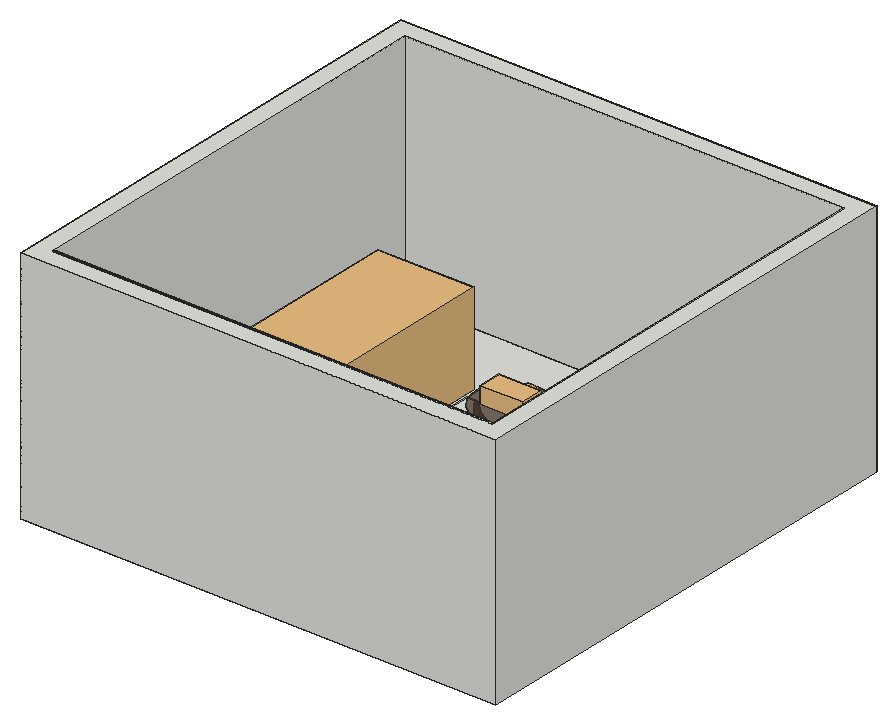
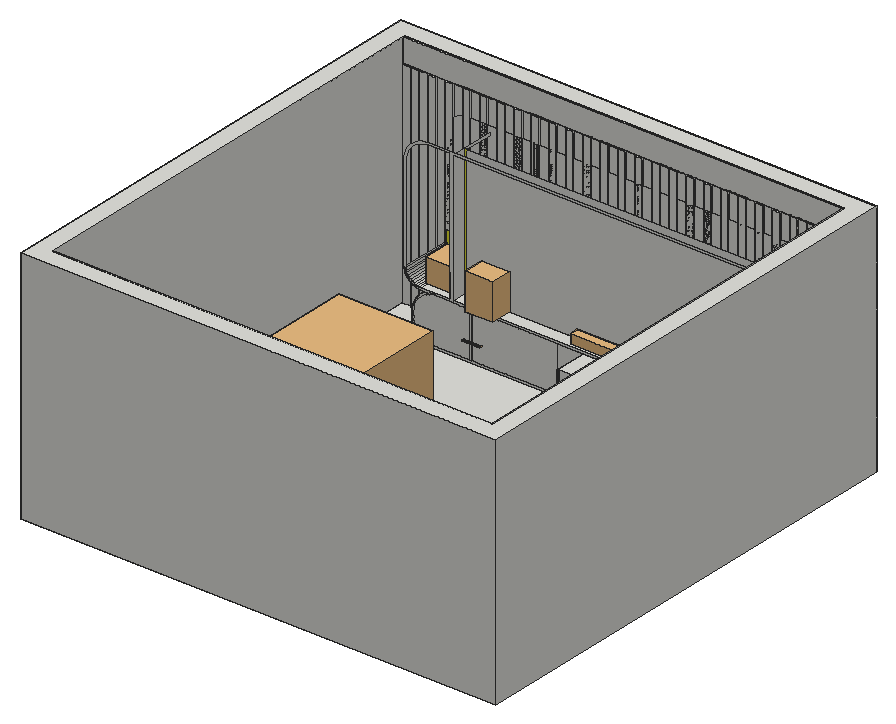
# SketchUp Ruby script. Lengths in inches.
U = 1.inch
M = Sketchup.active_model
def pt(a) = Geom::Point3d.new(a.map { |v| v * U })
def face(e, loops, mat)
  f = e.add_face(loops[0].map { |a| pt(a) })
  loops[1..].each { |l| e.add_face(l.map { |a| pt(a) }).erase! }
  f.material = f.back_material = mat if mat
  f
end
# faces: each face lists its corners as indices into pts; further lists are holes
def faces(e, pts, list, mat = nil) = list.each { |f| face(e, (f[0].is_a?(Array) ? f : [f]).map { |l| l.map { |i| pts[i] } }, mat) }
# xy, xz, yz: faces in a plane at the given z, y or x. An outline is a flat list of corners, or four numbers for a rectangle; further outlines are holes
def ring(l) = l.size == 4 ? [[l[0], l[1]], [l[2], l[1]], [l[2], l[3]], [l[0], l[3]]] : l.each_slice(2).to_a
def flat(e, list, mat, &to3) = list.each { |f| face(e, (f[0].is_a?(Array) ? f : [f]).map { |l| ring(l).map { |u, v| to3.(u, v) } }, mat) }
def xy(e, z, list, mat = nil) = flat(e, list, mat) { |x, y| [x, y, z] }
def xz(e, y, list, mat = nil) = flat(e, list, mat) { |x, z| [x, y, z] }
def yz(e, x, list, mat = nil) = flat(e, list, mat) { |y, z| [x, y, z] }
def lines(e, pts, list) = list.each { |a, b| e.add_line(pt(pts[a]), pt(pts[b])) }
# prism: a flat outline (further loops are holes) pulled along v
def prism(e, loops, v, mat = nil)
  f = face(e, loops, mat); d = Geom::Vector3d.new(v.map { |x| x * U })
  f.pushpull(f.normal.samedirection?(d) ? d.length : -d.length)
end
def box(e, o, s, mat = nil) = prism(e, [[o, [o[0] + s[0], o[1], o[2]], [o[0] + s[0], o[1] + s[1], o[2]], [o[0], o[1] + s[1], o[2]]]], [0, 0, s[2]], mat)
def at(x, y, z, deg = 0) = Geom::Transformation.translation(pt([x, y, z])) * Geom::Transformation.rotation(ORIGIN, Z_AXIS, deg.degrees)
def axes(o, x, y, z) = Geom::Transformation.new([*x, 0, *y, 0, *z, 0, *pt(o).to_a, 1])
def part(name) = M.definitions.add(name)
# library, detail: a bought-in or finely detailed component or shape, given as its bounding box
def library(name, o, s) = part(name).tap { |d| box(d.entities, o, s) }
def detail(e, o, s) = box(e.add_group.entities, o, s)
def put(e, d, t, mat = nil) = e.add_instance(d, t).tap { |i| i.material = mat if mat }
def group(e, t, mat = nil) = e.add_group.tap { |g| g.transformation = t; g.material = mat if mat }.entities
root = M.entities
M.materials.add("Color_D03").color = [255, 216, 101]
M.materials.add("Glass Dark").color = [71, 58, 43]
M.materials["Glass Dark"].alpha = 0.46
M.materials.add("[0134_DimGray]").color = [105, 105, 105]
M.materials.add("[0136_Charcoal]").color = [211, 185, 236]
M.materials.add("[Color G07]").color = [232, 230, 47]
M.materials.add("[Color M09]4").color = [0, 0, 0]
M.materials.add("notenhout").color = [99, 83, 84]
c1 = library("01",[0,0,0],[101.45,38.38,34.47])
c2 = library("Modern Round Tea Table",[0,0,0],[24.84,25.09,16.45])
c3 = part("Group\#19")
prism(c3.entities,[[[1.97,0,0],[1.97,39.37,0],[1.97,39.37,17.72],[1.97,37.14,17.72],[1.97,36.88,14.6875],[1.97,35.37,11.01],[1.97,32.79,7.79],[1.97,29.32,5.24],[1.97,25.19,3.54],[1.97,20.69,2.82],[1.97,16.12,3.1],[1.97,11.79,4.38],[1.97,8,6.58],[1.97,5.01,9.53],[1.97,3.01,13.03],[1.97,2.15,16.86],[1.97,2.23,17.72],[1.97,0,17.72]]],[-1.97,0,0],"notenhout")
c4 = part("japandi+table+glass+~")
g1 = group(c4.entities,at(26.82,84.01,17.85,-66.1))
prism(g1,[[[1.1875,15.62,0],[0,21.54,0],[0.38,27.57,0],[2.32,33.3,0],[5.67,38.33,0],[10.2,42.32,0],[15.62,45.01,0],[21.54,46.19,0],[27.57,45.81,0],[33.3,43.88,0],[38.33,40.53,0],[42.32,35.99,0],[45.01,30.58,0],[46.19,24.65,0],[45.81,18.62,0],[43.88,12.9,0],[40.53,7.86,0],[35.99,3.87,0],[30.58,1.1875,0],[24.65,0,0],[18.62,0.38,0],[12.9,2.32,0],[7.86,5.67,0],[3.87,10.2,0]]],[0,0,0.98],"Glass Dark")
put(c4.entities,c3,at(39.85,63.81,0,-66.1))
put(c4.entities,c3,at(50.43,90.37,0,-156.1))
c5 = part("232mm Slimline Handle")
detail(c5.entities,[0,0,0],[9.13,0.47,1.38])
c6 = part("skeF")
xy(c6.entities,0,[[0,0,50,36.34]])
xy(c6.entities,1.875,[[0,0,50,0,50,36.34,47.5,36.34,47.5,1.02,2.5,1.02,2.5,36.34,0,36.34]])
xy(c6.entities,2.8125,[[[2.5,1.02,47.5,6.25],[3.75,1.64,46.25,5.625]],[3.75,1.64,46.25,5.625]])
xy(c6.entities,3.75,[[[2.5,6.25,47.5,36.34],[5.625,9.375,44.375,33.125],[45.24,9.51,46.51,9.98],[45.24,11.8,46.51,12.27],[45.24,10.25,46.51,10.72],[45.24,10.99,46.51,11.46]],[5.625,9.375,44.375,33.125],[45.24,9.51,46.51,9.98],[45.24,10.25,46.51,10.72],[45.24,10.99,46.51,11.46],
  [45.24,11.8,46.51,12.27]])
xz(c6.entities,0,[[0,0,50,1.875]])
xz(c6.entities,1.02,[[2.5,1.875,47.5,2.8125]])
xz(c6.entities,6.25,[[2.5,2.8125,47.5,3.75]])
xz(c6.entities,36.34,[[0,0,50,1.875],[2.5,1.875,47.5,3.75]])
yz(c6.entities,0,[[0,0,36.34,1.875]])
yz(c6.entities,2.5,[[1.02,1.875,1.02,2.8125,6.25,2.8125,6.25,3.75,36.34,3.75,36.34,1.875]])
yz(c6.entities,47.5,[[1.02,1.875,36.34,1.875,36.34,3.75,6.25,3.75,6.25,2.8125,1.02,2.8125]])
yz(c6.entities,50,[[0,0,36.34,1.875]])
c7 = part("SONY\#1")
xy(c7.entities,0.02,[[1.44,0,1.15,0.02,0.9,0.07,0.68,0.16,0.51,0.28,0.375,0.43,0.27,0.6,0.21,0.79,0.19,1,0.5625,1,0.59,0.84,0.65,0.71,0.73,0.6,0.84,0.51,0.96,0.44,1.11,0.39,1.43,0.35,1.72,0.39,1.95,0.49,2.04,0.56,2.1,0.65,2.14,0.74,2.15,0.85,2.14,0.97,2.1,1.0625,2.04,1.14,1.95,1.21,1.67,1.32,1.23,1.43,0.8,1.55,0.64,1.63,0.51,1.72,0.41,1.83,0.34,1.95,0.3,2.08,0.29,2.23,0.31,2.4,0.36,2.56,0.45,2.7,0.57,2.82,0.73,2.92,0.91,2.99,1.11,3.04,1.34,3.05,1.57,3.04,1.79,2.99,1.98,2.92,2.14,2.82,2.28,2.69,2.375,2.54,2.4375,2.36,2.46,2.16,2.08,2.16,2.06,2.29,2.02,2.4,1.95,2.49,1.87,2.57,1.77,2.625,1.65,2.67,1.35,2.7,1.0625,2.67,0.85,2.58,0.77,2.51,0.71,2.43,0.68,2.35,0.67,2.25,0.7,2.09,0.8125,1.97,1.02,1.88,1.35,1.79,1.97,1.625,2.1875,1.52,2.37,1.36,2.44,1.26,2.49,1.15,2.52,1.03,2.54,0.88,2.52,0.7,2.46,0.54,2.36,0.39,2.23,0.25,2.07,0.14,1.88,0.0625,1.67,0.02],[[4.36,0,4.06,0.03,3.79,0.1,3.55,0.24,3.34,0.42,3.16,0.65,3.04,0.91,2.97,1.2,2.94,1.53,2.97,1.85,3.04,2.15,3.16,2.41,3.34,2.63,3.55,2.81,3.79,2.95,4.06,3.02,4.36,3.05,4.65,3.02,4.92,2.95,5.16,2.81,5.37,2.63,5.54,2.41,5.67,2.15,5.74,1.85,5.76,1.53,5.74,1.2,5.67,0.9,5.54,0.64,5.37,0.42,5.16,0.24,4.92,0.1,4.65,0.03],[4.35,0.33,4.5625,0.35,4.75,0.41,4.93,0.51,5.08,0.65,5.2,0.82,5.29,1.02,5.34,1.26,5.36,1.53,5.34,1.79,5.29,2.03,5.2,2.23,5.08,2.4,4.93,2.54,4.76,2.64,4.57,2.7,4.36,2.72,4.15,2.7,3.96,2.64,3.78,2.54,3.63,2.4,3.51,2.23,3.42,2.03,3.36,1.79,3.35,1.53,3.36,1.26,3.42,1.03,3.51,0.82,3.63,0.65,3.78,0.51,3.95,0.41,4.14,0.35]],[6.28,0.05,6.28,3,6.68,3,8.23,0.67,8.23,3,8.6,3,8.6,0.05,8.2,0.05,6.65,2.38,6.65,0.05],[10.11,0.05,10.11,1.3,8.95,3,9.42,3,10.31,1.64,11.18,3,11.66,3,10.5,1.3,10.5,0.05]])
c8 = part("Untitled (8)")
put(c8.entities,c6,at(36.34,-31.65,0),"Color_D03")
put(c8.entities,c7,at(55.46,-30.01,2.8125))
c9 = library("tasse",[17.31,42.26,0],[5.26,6.09,5.2])
c10 = library("Serving 10 ",[0,0,0],[18.76,10.8,8.42])
c11 = library("Panasonic+SC-HTB8+sound+bar",[0,-0.18,0],[29.53,4.33,2.36])
c12 = library("TV+remote",[138.89,58.58,0],[104.14,438.75,34])
c13 = library("Plant",[-15.17,-14.95,0],[35.27,31.45,46.14])
c14 = library("Buddha+++fountain+",[-17.29,-21.67,-1.59],[33.47,33.42,28.7])
c15 = library("Flower pot 12",[-12.91,-12.4,0],[25.81,25.8,45.6875])
xy(root,0,[[[0,0,240,240],[9,9,231,231]],[9,9,231,10],[[9,10,231,231],[76.664,81.343,148.977,185.781]],[13.856,11,204.943,12.6875]])
xy(root,0.1,[[76.664,81.343,148.977,185.781]])
xy(root,4,[[13.856,11,204.943,12.6875],[13.856,12.6875,204.943,37]])
xy(root,5,[[43.356,36.6,44.356,37],[87.051,36.6,88.051,36.788],[130.747,36.6,131.747,36.9],[174.443,36.6,175.443,37],[87.051,36.788,88.051,37],
  [130.747,36.9,131.747,37]])
xy(root,16.5,[[87.551,17,131.247,21],[87.551,21,88.051,36.6],[88.051,21,130.747,37],[130.747,21,131.247,36.6],[87.051,36.6,87.551,36.788],
  [87.551,36.6,88.051,36.788],[130.747,36.6,131.247,36.9],[131.247,36.6,131.747,36.9],[87.051,36.788,87.551,37],[131.247,36.9,131.747,37]])
xy(root,28,[[197.325,11,200.205,37],[87.551,17,131.247,21],[87.551,21,131.247,37],[43.356,36.6,44.356,37],[174.443,36.6,175.443,37]])
xy(root,29,[[26.356,11,204.189,11,204.189,37,200.205,37,200.205,11.1,185.773,11.1,185.773,37,183.773,37,183.773,30.3125,36.631,30.3125,36.631,26.3125,36.031,26.3125,36.031,30.3125,35.431,30.3125,35.431,26.3125,34.831,26.3125,34.831,30.3125,34.231,30.3125,34.231,26.3125,33.631,26.3125,33.631,30.3125,33.031,30.3125,33.031,26.3125,32.431,26.3125,32.431,30.3125,31.831,30.3125,31.831,26.3125,31.231,26.3125,31.231,30.3125,30.631,30.3125,30.631,26.3125,30.031,26.3125,30.031,30.3125,29.431,30.3125,29.431,26.375,28.831,26.375,28.831,30.3125,28.231,30.3125,28.231,26.375,27.631,26.375,27.631,30.3125,27.031,30.3125,27.031,26.375,26.431,26.375,26.431,30.3125,26.356,30.3125],[185.773,11.1,200.205,37],[24.079,15,24.231,30.3125],[30.031,26.3125,30.631,26.3125,30.631,30.3125,31.231,30.3125,31.231,26.3125,31.831,26.3125,31.831,30.3125,32.431,30.3125,32.431,26.3125,33.031,26.3125,33.031,30.3125,33.631,30.3125,33.631,26.3125,34.231,26.3125,34.231,30.3125,34.831,30.3125,34.831,26.3125,35.431,26.3125,35.431,30.3125,36.031,30.3125,36.031,26.3125,36.631,26.3125,36.631,30.3125,183.773,30.3125,183.773,37,24.079,37,24.079,30.3125,25.231,30.3125,25.231,26.375,25.831,26.375,25.831,30.3125,26.431,30.3125,26.431,26.375,27.031,26.375,27.031,30.3125,27.631,30.3125,27.631,26.375,28.231,26.375,28.231,30.3125,28.831,30.3125,28.831,26.375,29.431,26.375,29.431,30.3125,30.031,30.3125]])
xy(root,120,[[[0,0,240,240],[9,9,231,231]],[9,9,231,10]])
xz(root,0,[[0,0,240,120]])
xz(root,9,[[9,0,231,120]])
xz(root,10,[[13.856,0,13.856,108,9,108,9,120,231,120,231,0],[9,0,13.856,108]])
xz(root,11,[[13.856,0,204.943,4],[13.856,4,204.943,4,204.943,16.5,204.836,18.132,204.517,19.735,203.991,21.284,203.268,22.75,202.36,24.11,201.282,25.339,200.052,26.417,198.693,27.325,197.325,28,24.079,28,22.745,28.087,22.078,28.22,21.572,28.048,20.106,27.325,18.746,26.417,17.517,25.339,16.439,24.11,15.531,22.75,14.807,21.284,14.282,19.735,13.963,18.132,13.856,16.5],[13.856,16.5,13.856,29,19.717,29,20.167,28.778,21.433,28.348,22.078,28.22,21.572,28.048,20.106,27.325,18.746,26.417,17.517,25.339,16.439,24.11,15.531,22.75,14.807,21.284,14.282,19.735,13.963,18.132],[24.079,28,200.205,28,201.324,28.073,202.423,28.292,203.484,28.652,204.189,29,26.356,29,24.724,28.893,23.121,28.574,22.078,28.22,22.745,28.087],[22.078,28.22,21.433,28.348,20.167,28.778,19.717,29,26.356,29,24.724,28.893,23.121,28.574],
  [19.717,29,204.189,29,204.489,29.148,205.421,29.77,206.263,30.509,207.002,31.352,207.625,32.284,208.12,33.289,208.481,34.35,208.699,35.449,208.773,36.567,208.773,83.69,208.667,85.297,208.353,86.876,207.836,88.401,207.123,89.845,206.229,91.184,205.167,92.395,203.957,93.456,202.618,94.351,201.174,95.063,199.649,95.581,198.07,95.895,196.463,96,25.222,96,23.738,95.903,22.28,95.613,20.872,95.135,19.539,94.477,18.303,93.651,17.185,92.671,16.205,91.553,15.379,90.317,14.721,88.984,14.243,87.576,13.953,86.117,13.856,84.634,13.856,38.224,13.943,36.889,14.204,35.577,14.634,34.311,15.226,33.112,15.969,32,16.85,30.994,17.856,30.113,18.968,29.37]])
xz(root,11.1,[[184.912,28.491,184.912,40.591,185.773,40.591,185.773,29,200.205,29,201.193,29.065,202.164,29.258,203.101,29.576,203.608,29.826,203.128,29.505,202.24,29.067,201.303,28.749,200.332,28.556,199.344,28.491],[185.773,29,185.773,40.591,206.912,40.591,206.912,36.059,206.847,35.071,206.654,34.1,206.336,33.163,205.898,32.275,205.348,31.452,204.695,30.708,203.951,30.055,203.608,29.826,203.101,29.576,202.164,29.258,201.193,29.065,200.205,29]])
xz(root,11.1,[[203.608,29.826,203.951,30.055,204.695,30.708,205.348,31.452,205.898,32.275,206.336,33.163,206.654,34.1,206.847,35.071,206.912,36.059,206.912,40.591,185.773,40.591,185.773,41.1,207.773,41.1,207.773,36.567,207.708,35.58,207.515,34.609,207.197,33.671,206.759,32.784,206.209,31.961,205.556,31.216,204.812,30.564,203.989,30.014]],"[Color G07]")
xz(root,12.6875,[[13.856,0,13.856,4,14.088,4,14.088,2.5,204.943,2.5,204.943,0]])
xz(root,12.6875,[[14.088,2.5,204.943,4]],"[0136_Charcoal]")
xz(root,17,[[87.551,16.5,131.247,28]])
xz(root,21,[[87.551,16.5,131.247,28]])
xz(root,26.3125,[[30.031,29,30.031,85.939,30.631,86.018,30.631,29],[31.231,29,31.231,86.097,31.831,86.018,31.831,29],[32.431,29,32.431,85.939,32.784,85.893,33.031,85.79,33.031,29],[33.631,29,33.631,85.542,34.231,85.293,34.231,29],[34.831,29,34.831,84.833,35.431,84.373,35.431,29],
  [36.031,29,36.031,83.614,36.427,83.097,36.631,82.605,36.631,29]])
xz(root,26.375,[[25.231,29,25.231,80.097,25.435,81.65,25.831,82.605,25.831,29],[26.431,29,26.431,83.614,26.988,84.34,27.031,84.373,27.031,29],[27.631,29,27.631,84.833,28.231,85.293,28.231,29],[28.831,29,28.831,85.542,29.431,85.79,29.431,29]])
xz(root,30.3125,[[38.231,29,38.231,80.163,38.001,81.911,37.555,82.988,37.301,83.602,36.824,84.222,36.187,85.053,36.04,85.166,35.44,85.626,34.735,86.167,34.014,86.466,33.414,86.714,33.045,86.867,32.561,86.931,31.961,87.01,31.231,87.106,30.5,87.01,29.9,86.931,29.417,86.867,29.048,86.714,28.448,86.466,27.727,86.167,27.022,85.626,26.422,85.166,26.275,85.053,25.638,84.222,25.161,83.602,24.907,82.988,24.461,81.911,24.231,80.163,24.231,29.056,23.875,29.079,22.692,29.314,21.55,29.702,20.468,30.236,19.464,30.906,18.557,31.702,17.762,32.609,17.092,33.612,16.558,34.694,16.17,35.836,15.935,37.02,15.856,38.224,15.856,84.634,15.945,85.987,16.209,87.317,16.645,88.601,17.245,89.817,17.998,90.944,18.892,91.964,19.912,92.858,21.039,93.611,22.255,94.211,23.539,94.647,24.869,94.911,26.218,95,26.222,95,180.896,94.958,181.991,94.958,182.164,94.866,182.339,94.731,182.489,94.57,182.61,94.385,182.7,94.184,182.754,93.97,182.773,93.75,182.773,29],[24.231,29,24.231,29.056,25.079,29],[25.079,29,24.231,29.056,24.231,80.163,24.461,81.911,24.907,82.988,25.161,83.602,25.638,84.222,26.275,85.053,26.422,85.166,27.022,85.626,27.727,86.167,28.448,86.466,29.048,86.714,29.417,86.867,29.9,86.931,30.5,87.01,31.231,87.106,31.961,87.01,32.561,86.931,33.045,86.867,33.414,86.714,34.014,86.466,34.735,86.167,35.44,85.626,36.04,85.166,36.187,85.053,36.824,84.222,37.301,83.602,37.555,82.988,38.001,81.911,38.231,80.163,38.231,29,37.231,29,37.231,80.097,37.026,81.65,36.631,82.605,36.427,83.097,36.031,83.614,35.474,84.34,35.431,84.373,34.231,85.293,33.631,85.542,33.031,85.79,32.784,85.893,32.431,85.939,31.231,86.097,30.031,85.939,29.678,85.893,29.431,85.79,28.831,85.542,28.231,85.293,27.031,84.373,26.988,84.34,26.431,83.614,26.035,83.097,25.831,82.605,25.435,81.65,25.231,80.097,25.231,29],[25.831,29,25.831,82.605,26.035,83.097,26.431,83.614,26.431,29],[27.031,29,27.031,84.373,27.631,84.833,27.631,29],
  [28.231,29,28.231,85.293,28.831,85.542,28.831,29],[29.431,29,29.431,85.79,29.678,85.893,30.031,85.939,30.031,29],[30.631,29,30.631,86.018,31.231,86.097,31.231,29],[31.831,29,31.831,86.018,32.431,85.939,32.431,29],[33.031,29,33.031,85.79,33.631,85.542,33.631,29],
  [34.231,29,34.231,85.293,34.831,84.833,34.831,29],[35.431,29,35.431,84.373,35.474,84.34,36.031,83.614,36.031,29],[36.631,29,36.631,82.605,37.026,81.65,37.231,80.097,37.231,29]])
xz(root,30.3125,[[24.079,29,22.875,29.079,21.692,29.314,20.55,29.702,19.468,30.236,18.464,30.906,17.557,31.702,16.762,32.609,16.092,33.612,15.558,34.694,15.17,35.836,14.935,37.02,14.856,38.224,14.856,84.634,14.945,85.987,15.209,87.317,15.645,88.601,16.245,89.817,16.998,90.944,17.892,91.964,18.912,92.858,20.039,93.611,21.255,94.211,22.539,94.647,23.869,94.911,25.222,95,26.218,95,24.869,94.911,23.539,94.647,22.255,94.211,21.039,93.611,19.912,92.858,18.892,91.964,17.998,90.944,17.245,89.817,16.645,88.601,16.209,87.317,15.945,85.987,15.856,84.634,15.856,38.224,15.935,37.02,16.17,35.836,16.558,34.694,17.092,33.612,17.762,32.609,18.557,31.702,19.464,30.906,20.468,30.236,21.55,29.702,22.692,29.314,23.875,29.079,24.231,29.056,24.231,29],[182.773,29,182.773,93.75,182.754,93.97,182.7,94.184,182.61,94.385,182.489,94.57,182.339,94.731,182.164,94.866,181.991,94.958,182.846,94.957,183.001,94.905,183.148,94.833,183.283,94.742,183.406,94.634,183.514,94.511,183.605,94.375,183.677,94.228,183.73,94.073,183.762,93.913,183.773,93.75,183.773,29]],"[Color G07]")
xz(root,36.6,[[87.051,5,88.051,16.5],[130.747,5,131.747,16.5]])
xz(root,36.6,[[43.356,5,44.356,28],[174.443,5,175.443,28]],"[Color M09]4")
xz(root,36.788,[[87.051,5,88.051,16.5]],"[Color M09]4")
xz(root,36.9,[[130.747,5,131.747,16.5]],"[Color M09]4")
xz(root,37,[[[13.856,4,13.856,16.5,13.963,18.132,14.282,19.735,14.807,21.284,15.531,22.75,16.439,24.11,17.517,25.339,18.746,26.417,20.106,27.325,21.572,28.048,22.078,28.22,21.433,28.348,20.167,28.778,18.968,29.37,17.856,30.113,16.85,30.994,15.969,32,15.226,33.112,14.634,34.311,14.204,35.577,13.943,36.889,13.856,38.224,13.856,84.634,13.953,86.117,14.243,87.576,14.721,88.984,15.379,90.317,16.205,91.553,17.185,92.671,18.303,93.651,19.539,94.477,20.872,95.135,22.28,95.613,23.738,95.903,25.222,96,196.463,96,198.07,95.895,199.649,95.581,201.174,95.063,202.618,94.351,203.957,93.456,205.167,92.395,206.229,91.184,207.123,89.845,207.836,88.401,208.353,86.876,208.667,85.297,208.773,83.69,208.773,36.567,208.699,35.449,208.481,34.35,208.12,33.289,207.625,32.284,207.002,31.352,206.263,30.509,205.421,29.77,204.489,29.148,204.189,29,200.205,29,201.193,29.065,202.164,29.258,203.101,29.576,203.989,30.014,204.812,30.564,205.556,31.216,206.209,31.961,206.759,32.784,207.197,33.671,207.515,34.609,207.708,35.58,207.773,36.567,207.773,83.69,207.676,85.167,207.387,86.618,206.912,88.018,206.257,89.345,205.435,90.575,204.46,91.6875,203.348,92.663,202.118,93.485,200.791,94.139,199.39,94.615,197.939,94.903,196.463,95,185.773,95,185.773,29,192.443,29,194.074,28.893,195.678,28.574,197.226,28.048,197.325,28,26.356,28,24.855,27.902,23.379,27.608,21.955,27.125,20.606,26.459,19.355,25.624,18.224,24.632,17.232,23.501,16.397,22.25,15.731,20.901,15.248,19.476,14.954,18.001,14.856,16.5,14.856,5,203.943,5,203.943,16.5,203.844,18.001,203.551,19.476,203.067,20.901,202.402,22.25,201.566,23.501,200.574,24.632,199.443,25.624,198.193,26.459,196.844,27.125,195.419,27.608,193.944,27.902,192.443,28,197.325,28,198.693,27.325,200.052,26.417,201.282,25.339,202.36,24.11,203.268,22.75,203.991,21.284,204.517,19.735,204.836,18.132,204.943,16.5,204.943,4],[24.079,29,183.773,29,183.773,95,25.222,95,23.869,94.911,22.539,94.647,21.255,94.211,20.039,93.611,18.912,92.858,17.892,91.964,16.998,90.944,16.245,89.817,15.645,88.601,15.209,87.317,14.945,85.987,14.856,84.634,14.856,38.224,14.935,37.02,15.17,35.836,15.558,34.694,16.092,33.612,16.762,32.609,17.557,31.702,18.464,30.906,19.468,30.236,20.55,29.702,21.692,29.314,22.875,29.079]],[14.856,5,14.856,16.5,14.954,18.001,15.248,19.476,15.731,20.901,16.397,22.25,17.232,23.501,18.224,24.632,19.355,25.624,20.606,26.459,21.955,27.125,23.379,27.608,24.855,27.902,26.356,28,43.356,28,43.356,5],[44.356,5,44.356,28,87.551,28,87.551,16.5,87.051,16.5,87.051,5],[88.051,5,130.747,16.5],[131.747,5,131.747,16.5,131.247,16.5,131.247,28,174.443,28,174.443,5],
  [175.443,5,175.443,28,192.443,28,193.944,27.902,195.419,27.608,196.844,27.125,198.193,26.459,199.443,25.624,200.574,24.632,201.566,23.501,202.402,22.25,203.067,20.901,203.551,19.476,203.844,18.001,203.943,16.5,203.943,5],[197.325,28,197.226,28.048,195.678,28.574,194.074,28.893,192.443,29,204.189,29,203.484,28.652,202.423,28.292,201.324,28.073,200.205,28]])
xz(root,81.343,[[76.664,0,148.977,0.1]])
xz(root,185.781,[[76.664,0,148.977,0.1]])
xz(root,231,[[9,0,231,120]])
xz(root,240,[[0,0,240,120]])
yz(root,0,[[0,0,240,120]])
yz(root,9,[[9,0,10,120],[9,0,231,120]])
yz(root,13.856,[[11,0,12.6875,4],[11,4,37,16.5]])
yz(root,24.231,[[15,29,30.3125,38.224]])
yz(root,25.231,[[26.375,29,30.3125,38.224]])
yz(root,25.831,[[26.375,29,30.3125,38.224]])
yz(root,26.431,[[26.375,29,30.3125,38.224]])
yz(root,27.031,[[26.375,29,30.3125,38.224]])
yz(root,27.631,[[26.375,29,30.3125,38.224]])
yz(root,28.231,[[26.375,29,30.3125,38.224]])
yz(root,28.831,[[26.375,29,30.3125,38.224]])
yz(root,29.431,[[26.375,29,30.3125,38.224]])
yz(root,30.031,[[26.3125,29,30.3125,38.224]])
yz(root,30.631,[[26.3125,29,30.3125,38.224]])
yz(root,31.231,[[26.3125,29,30.3125,38.224]])
yz(root,31.831,[[26.3125,29,30.3125,38.224]])
yz(root,32.431,[[26.3125,29,30.3125,38.224]])
yz(root,33.031,[[26.3125,29,30.3125,38.224]])
yz(root,33.631,[[26.3125,29,30.3125,38.224]])
yz(root,34.231,[[26.3125,29,30.3125,38.224]])
yz(root,34.831,[[26.3125,29,30.3125,38.224]])
yz(root,35.431,[[26.3125,29,30.3125,38.224]])
yz(root,36.031,[[26.3125,29,30.3125,38.224]])
yz(root,36.631,[[26.3125,29,30.3125,38.224]])
yz(root,38.231,[[15,29,30.3125,38.224]])
yz(root,43.356,[[36.6,5,37,28]])
yz(root,44.356,[[36.6,5,37,28]])
yz(root,76.664,[[81.343,0,185.781,0.1]])
yz(root,87.051,[[36.6,5,36.788,16.5],[36.788,5,37,16.5]])
yz(root,87.551,[[17,16.5,21,28],[21,16.5,37,28]])
yz(root,88.051,[[36.6,5,36.788,16.5],[36.788,5,37,16.5]])
yz(root,130.747,[[36.6,5,36.9,16.5],[36.9,5,37,16.5]])
yz(root,131.247,[[17,16.5,21,28],[21,16.5,37,28]])
yz(root,131.747,[[36.6,5,36.9,16.5],[36.9,5,37,16.5]])
yz(root,148.977,[[81.343,0,185.781,0.1]])
yz(root,174.443,[[36.6,5,37,28]])
yz(root,175.443,[[36.6,5,37,28]])
yz(root,183.773,[[30.3125,29,30.3125,93.75,14.3125,93.75,14.3125,95,37,95,37,29]])
yz(root,185.773,[[11.1,29,37,41.1]])
yz(root,204.943,[[11,0,12.6875,4],[11,4,37,16.5]])
yz(root,231,[[9,0,10,120],[10,0,231,120]])
yz(root,240,[[0,0,240,120]])
p = [[13.963,37,18.132],[13.856,37,16.5],[13.856,11,16.5],[13.963,11,18.132],[204.943,37,16.5],[204.836,37,18.132],
  [204.836,11,18.132],[204.943,11,16.5],[14.282,37,19.735],[14.282,11,19.735],[204.517,37,19.735],[204.517,11,19.735],
  [14.807,37,21.284],[14.807,11,21.284],[203.991,37,21.284],[203.991,11,21.284],[15.531,37,22.75],[15.531,11,22.75],
  [203.268,37,22.75],[203.268,11,22.75],[16.439,37,24.11],[16.439,11,24.11],[202.36,37,24.11],[202.36,11,24.11],
  [17.517,37,25.339],[17.517,11,25.339],[201.282,37,25.339],[201.282,11,25.339],[18.746,37,26.417],[18.746,11,26.417],
  [200.052,37,26.417],[200.052,11,26.417],[20.106,37,27.325],[20.106,11,27.325],[198.693,37,27.325],[198.693,11,27.325],
  [21.572,37,28.048],[21.572,11,28.048],[197.325,37,28],[197.325,11,28],[22.078,37,28.22],[22.078,11,28.22],
  [23.121,11,28.574],[23.121,37,28.574],[200.205,11,28],[200.205,37,28],[201.324,37,28.073],[201.324,11,28.073],
  [202.423,37,28.292],[202.423,11,28.292],[21.433,11,28.348],[20.167,11,28.778],[20.167,37,28.778],[21.433,37,28.348],
  [203.484,37,28.652],[203.484,11,28.652],[24.724,37,28.893],[24.724,11,28.893],[204.189,37,29],[204.189,11,29],
  [19.717,11,29],[18.968,11,29.37],[18.968,37,29.37],[204.489,11,29.148],[204.489,37,29.148],[201.193,11.1,29.065],
  [201.193,37,29.065],[200.205,37,29],[200.205,11.1,29],[22.875,15,29.079],[24.079,15,29],[24.079,30.3125,29],
  [22.875,30.3125,29.079],[22.875,37,29.079],[24.079,37,29],[205.421,37,29.77],[205.421,11,29.77],[202.164,11.1,29.258],
  [202.164,37,29.258],[21.692,15,29.314],[21.692,30.3125,29.314],[21.692,37,29.314],[203.101,11.1,29.576],[203.101,37,29.576],
  [20.55,15,29.702],[20.55,30.3125,29.702],[20.55,37,29.702],[17.856,11,30.113],[17.856,37,30.113],[203.989,11.1,30.014],
  [203.989,37,30.014],[203.608,11.1,29.826],[19.468,15,30.236],[19.468,30.3125,30.236],[19.468,37,30.236],[206.263,37,30.509],
  [206.263,11,30.509],[204.812,11.1,30.564],[204.812,37,30.564],[16.85,11,30.994],[16.85,37,30.994],[18.464,15,30.906],
  [18.464,30.3125,30.906],[18.464,37,30.906],[207.002,37,31.352],[207.002,11,31.352],[205.556,11.1,31.216],[205.556,37,31.216],
  [17.557,15,31.702],[17.557,30.3125,31.702],[17.557,37,31.702],[15.969,11,32],[15.969,37,32],[206.209,11.1,31.961],
  [206.209,37,31.961],[207.625,37,32.284],[207.625,11,32.284],[16.762,15,32.609],[16.762,30.3125,32.609],[16.762,37,32.609],
  [15.226,11,33.112],[15.226,37,33.112],[206.759,11.1,32.784],[206.759,37,32.784],[208.12,37,33.289],[208.12,11,33.289],
  [16.092,15,33.612],[16.092,30.3125,33.612],[16.092,37,33.612],[207.197,11.1,33.671],[207.197,37,33.671],[14.634,11,34.311],
  [14.634,37,34.311],[208.481,37,34.35],[208.481,11,34.35],[15.558,15,34.694],[15.558,30.3125,34.694],[15.558,37,34.694],
  [207.515,11.1,34.609],[207.515,37,34.609],[14.204,11,35.577],[14.204,37,35.577],[208.699,37,35.449],[208.699,11,35.449],
  [207.708,11.1,35.58],[207.708,37,35.58],[15.17,15,35.836],[15.17,30.3125,35.836],[15.17,37,35.836],[24.079,11,28],
  [24.079,37,28],[26.356,37,29]]
faces(root,p,[[0,1,2,3],[4,5,6,7],[8,0,3,9],[5,10,11,6],[12,8,9,13],[10,14,15,11],[16,12,13,17],[14,18,19,15],
  [20,16,17,21],[18,22,23,19],[24,20,21,25],[22,26,27,23],[28,24,25,29],[26,30,31,27],[32,28,29,33],[30,34,35,31],
  [36,32,33,37],[34,38,39,35],[40,36,37,41,42,43],[44,45,46,47],[47,46,48,49],[50,51,52,53],[49,48,54,55],[56,43,42,57],
  [55,54,58,59],[60,61,62,52,51],[63,59,58,64],[65,66,67,68],[69,70,71,72],[73,72,71,74],[63,64,75,76],[77,78,66,65],
  [79,69,72,80],[81,80,72,73],[82,83,78,77],[84,79,80,85],[86,85,80,81],[61,87,88,62],[89,90,83,82,91],[92,84,85,93],
  [94,93,85,86],[76,75,95,96],[97,98,90,89],[87,99,100,88],[101,92,93,102],[103,102,93,94],[96,95,104,105],[106,107,98,97],
  [108,101,102,109],[110,109,102,103],[99,111,112,100],[113,114,107,106],[105,104,115,116],[117,108,109,118],[119,118,109,110],[111,120,121,112],
  [122,123,114,113],[116,115,124,125],[126,117,118,127],[128,127,118,119],[129,130,123,122],[120,131,132,121],[125,124,133,134],[135,126,127,136],
  [137,136,127,128],[138,139,130,129],[131,140,141,132],[134,133,142,143],[144,145,139,138],[146,135,136,147],[148,147,136,137]])
lines(root,p,[[149,150],[56,151]])
put(root,c1,axes([200.0625,89.15,0],[0,1,0],[-1.24,0,0],[0,0,1.43]))
put(root,c1,axes([26.27,192.53,0],[0,-1,0],[1.26,0,0],[0,0,1.34]))
g2 = group(root,at(9,10,0))
xy(g2,0,[[0,0,4.86,0.5],[4.86,0,8.6875,1],[8.6875,0,13.54,0.5],[13.54,0,17.37,1],[17.37,0,22.23,0.5],
  [22.23,0,26.06,1],[26.06,0,30.91,0.5],[30.91,0,34.74,1],[34.74,0,39.6,0.5],[39.6,0,43.43,1],
  [43.43,0,48.28,0.5],[48.28,0,52.11,1],[52.11,0,56.97,0.5],[56.97,0,60.8,1],[60.8,0,65.66,0.5],
  [65.66,0,69.49,1],[69.49,0,74.34,0.5],[74.34,0,78.17,1],[78.17,0,83.03,0.5],[83.03,0,86.86,1],
  [86.86,0,91.71,0.5],[91.71,0,95.54,1],[95.54,0,100.4,0.5],[100.4,0,104.23,1],[104.23,0,109.09,0.5],
  [109.09,0,112.91,1],[112.91,0,117.77,0.5],[117.77,0,121.6,1],[121.6,0,126.46,0.5],[126.46,0,130.29,1],
  [130.29,0,135.14,0.5],[135.14,0,138.97,1],[138.97,0,143.83,0.5],[143.83,0,147.66,1],[147.66,0,152.51,0.5],
  [152.51,0,156.34,1],[156.34,0,161.2,0.5],[161.2,0,165.03,1],[165.03,0,169.89,0.5],[169.89,0,173.72,1],
  [173.72,0,178.57,0.5],[178.57,0,182.4,1],[182.4,0,187.26,0.5],[187.26,0,191.09,1],[191.09,0,195.94,0.5],
  [195.94,0,199.77,1],[199.77,0,204.63,0.5],[204.63,0,208.46,1],[208.46,0,213.3125,0.5],[213.3125,0,217.14,1],
  [217.14,0,222,0.5]])
xy(g2,108,[[0,0,4.86,0.5],[4.86,0,8.6875,1],[8.6875,0,13.54,0.5],[13.54,0,17.37,1],[17.37,0,22.23,0.5],
  [22.23,0,26.06,1],[26.06,0,30.91,0.5],[30.91,0,34.74,1],[34.74,0,39.6,0.5],[39.6,0,43.43,1],
  [43.43,0,48.28,0.5],[48.28,0,52.11,1],[52.11,0,56.97,0.5],[56.97,0,60.8,1],[60.8,0,65.66,0.5],
  [65.66,0,69.49,1],[69.49,0,74.34,0.5],[74.34,0,78.17,1],[78.17,0,83.03,0.5],[83.03,0,86.86,1],
  [86.86,0,91.71,0.5],[91.71,0,95.54,1],[95.54,0,100.4,0.5],[100.4,0,104.23,1],[104.23,0,109.09,0.5],
  [109.09,0,112.91,1],[112.91,0,117.77,0.5],[117.77,0,121.6,1],[121.6,0,126.46,0.5],[126.46,0,130.29,1],
  [130.29,0,135.14,0.5],[135.14,0,138.97,1],[138.97,0,143.83,0.5],[143.83,0,147.66,1],[147.66,0,152.51,0.5],
  [152.51,0,156.34,1],[156.34,0,161.2,0.5],[161.2,0,165.03,1],[165.03,0,169.89,0.5],[169.89,0,173.72,1],
  [173.72,0,178.57,0.5],[178.57,0,182.4,1],[182.4,0,187.26,0.5],[187.26,0,191.09,1],[191.09,0,195.94,0.5],
  [195.94,0,199.77,1],[199.77,0,204.63,0.5],[204.63,0,208.46,1],[208.46,0,213.3125,0.5],[213.3125,0,217.14,1],
  [217.14,0,222,0.5]])
xz(g2,0,[[0,0,4.86,108],[4.86,0,8.6875,108],[8.6875,0,13.54,108],[13.54,0,17.37,108],[17.37,0,22.23,108],
  [22.23,0,26.06,108],[26.06,0,30.91,108],[30.91,0,34.74,108],[34.74,0,39.6,108],[39.6,0,43.43,108],
  [43.43,0,48.28,108],[48.28,0,52.11,108],[52.11,0,56.97,108],[56.97,0,60.8,108],[60.8,0,65.66,108],
  [65.66,0,69.49,108],[69.49,0,74.34,108],[74.34,0,78.17,108],[78.17,0,83.03,108],[83.03,0,86.86,108],
  [86.86,0,91.71,108],[91.71,0,95.54,108],[95.54,0,100.4,108],[100.4,0,104.23,108],[104.23,0,109.09,108],
  [109.09,0,112.91,108],[112.91,0,117.77,108],[117.77,0,121.6,108],[121.6,0,126.46,108],[126.46,0,130.29,108],
  [130.29,0,135.14,108],[135.14,0,138.97,108],[138.97,0,143.83,108],[143.83,0,147.66,108],[147.66,0,152.51,108],
  [152.51,0,156.34,108],[156.34,0,161.2,108],[161.2,0,165.03,108],[165.03,0,169.89,108],[169.89,0,173.72,108],
  [173.72,0,178.57,108],[178.57,0,182.4,108],[182.4,0,187.26,108],[187.26,0,191.09,108],[191.09,0,195.94,108],
  [195.94,0,199.77,108],[199.77,0,204.63,108],[204.63,0,208.46,108],[208.46,0,213.3125,108],[213.3125,0,217.14,108],
  [217.14,0,222,108]])
xz(g2,0.5,[[0,0,4.86,108],[8.6875,0,13.54,108],[17.37,0,22.23,108],[26.06,0,30.91,108],[34.74,0,39.6,108],
  [43.43,0,48.28,108],[52.11,0,56.97,108],[60.8,0,65.66,108],[69.49,0,74.34,108],[78.17,0,83.03,108],
  [86.86,0,91.71,108],[95.54,0,100.4,108],[104.23,0,109.09,108],[112.91,0,117.77,108],[121.6,0,126.46,108],
  [130.29,0,135.14,108],[138.97,0,143.83,108],[147.66,0,152.51,108],[156.34,0,161.2,108],[165.03,0,169.89,108],
  [173.72,0,178.57,108],[182.4,0,187.26,108],[191.09,0,195.94,108],[199.77,0,204.63,108],[208.46,0,213.3125,108],
  [217.14,0,222,108]])
xz(g2,1,[[4.86,0,8.6875,108],[13.54,0,17.37,108],[22.23,0,26.06,108],[30.91,0,34.74,108],[39.6,0,43.43,108],
  [48.28,0,52.11,108],[56.97,0,60.8,108],[65.66,0,69.49,108],[74.34,0,78.17,108],[83.03,0,86.86,108],
  [91.71,0,95.54,108],[100.4,0,104.23,108],[109.09,0,112.91,108],[117.77,0,121.6,108],[126.46,0,130.29,108],
  [135.14,0,138.97,108],[143.83,0,147.66,108],[152.51,0,156.34,108],[161.2,0,165.03,108],[169.89,0,173.72,108],
  [178.57,0,182.4,108],[187.26,0,191.09,108],[195.94,0,199.77,108],[204.63,0,208.46,108],[213.3125,0,217.14,108]])
yz(g2,0,[[0,0,0.5,108]])
yz(g2,4.86,[[0,0,0.5,108],[0.5,0,1,108]])
yz(g2,8.6875,[[0.5,0,1,108]])
yz(g2,13.54,[[0,0,0.5,108],[0.5,0,1,108]])
yz(g2,17.37,[[0.5,0,1,108]])
yz(g2,22.23,[[0,0,0.5,108],[0.5,0,1,108]])
yz(g2,26.06,[[0.5,0,1,108]])
yz(g2,30.91,[[0,0,0.5,108],[0.5,0,1,108]])
yz(g2,34.74,[[0.5,0,1,108]])
yz(g2,39.6,[[0,0,0.5,108],[0.5,0,1,108]])
yz(g2,43.43,[[0.5,0,1,108]])
yz(g2,48.28,[[0,0,0.5,108],[0.5,0,1,108]])
yz(g2,52.11,[[0.5,0,1,108]])
yz(g2,56.97,[[0,0,0.5,108],[0.5,0,1,108]])
yz(g2,60.8,[[0.5,0,1,108]])
yz(g2,65.66,[[0,0,0.5,108],[0.5,0,1,108]])
yz(g2,69.49,[[0.5,0,1,108]])
yz(g2,74.34,[[0,0,0.5,108],[0.5,0,1,108]])
yz(g2,78.17,[[0.5,0,1,108]])
yz(g2,83.03,[[0,0,0.5,108],[0.5,0,1,108]])
yz(g2,86.86,[[0.5,0,1,108]])
yz(g2,91.71,[[0,0,0.5,108],[0.5,0,1,108]])
yz(g2,95.54,[[0.5,0,1,108]])
yz(g2,100.4,[[0,0,0.5,108],[0.5,0,1,108]])
yz(g2,104.23,[[0.5,0,1,108]])
yz(g2,109.09,[[0,0,0.5,108],[0.5,0,1,108]])
yz(g2,112.91,[[0.5,0,1,108]])
yz(g2,117.77,[[0,0,0.5,108],[0.5,0,1,108]])
yz(g2,121.6,[[0.5,0,1,108]])
yz(g2,126.46,[[0,0,0.5,108],[0.5,0,1,108]])
yz(g2,130.29,[[0.5,0,1,108]])
yz(g2,135.14,[[0,0,0.5,108],[0.5,0,1,108]])
yz(g2,138.97,[[0.5,0,1,108]])
yz(g2,143.83,[[0,0,0.5,108],[0.5,0,1,108]])
yz(g2,147.66,[[0.5,0,1,108]])
yz(g2,152.51,[[0,0,0.5,108],[0.5,0,1,108]])
yz(g2,156.34,[[0.5,0,1,108]])
yz(g2,161.2,[[0,0,0.5,108],[0.5,0,1,108]])
yz(g2,165.03,[[0.5,0,1,108]])
yz(g2,169.89,[[0,0,0.5,108],[0.5,0,1,108]])
yz(g2,173.72,[[0.5,0,1,108]])
yz(g2,178.57,[[0,0,0.5,108],[0.5,0,1,108]])
yz(g2,182.4,[[0.5,0,1,108]])
yz(g2,187.26,[[0,0,0.5,108],[0.5,0,1,108]])
yz(g2,191.09,[[0.5,0,1,108]])
yz(g2,195.94,[[0,0,0.5,108],[0.5,0,1,108]])
yz(g2,199.77,[[0.5,0,1,108]])
yz(g2,204.63,[[0,0,0.5,108],[0.5,0,1,108]])
yz(g2,208.46,[[0.5,0,1,108]])
yz(g2,213.3125,[[0,0,0.5,108],[0.5,0,1,108]])
yz(g2,217.14,[[0.5,0,1,108]])
yz(g2,222,[[0,0,0.5,108]])
put(root,c2,axes([95.26,97.37,0],[1.17,0,0],[0,1.2,0],[0,0,1.16]))
put(root,c4,axes([70.46,110.51,4.27],[0.7735,0,0],[0,0.7735,0],[0,0,0.7735]))
put(root,c5,axes([178.64,37,13.18],[-1,0,0],[0,0,1],[0,1,0]),"[Color M09]4")
put(root,c5,axes([48.95,37,15.25],[-1,0,0],[0,0,1],[0,1,0]),"[Color M09]4")
put(root,c8,axes([128.33,25.13,16.5],[-0.31,0,0],[0,-0.31,0],[0,0,0.31]))
put(root,c9,at(97,128.91,18.6))
put(root,c9,at(92.52,66.22,18.6))
put(root,c10,axes([105.07,158.63,18.83],[1.14,0,0],[0,1.1,0],[0,0,1]))
put(root,c11,axes([126.12,35.1875,29],[-1.22,0,0],[0,-1,0],[0,0,2]),"[0134_DimGray]")
put(root,c12,axes([62.46,30.62,29],[0,0.02625,0],[0.02625,0,0],[0,0,0.02625]))
put(root,c13,axes([166.81,34.25,29],[0.39712,0,0],[0,0.39712,0],[0,0,0.39712]))
put(root,c14,axes([194.16,23.9375,29.66],[-0.41272,0,0],[0,-0.41272,0],[0,0,0.41272]))
put(root,c15,axes([43.62,33.96,29.17],[0.24,0,0],[0,0.24,0],[0,0,0.24]))
